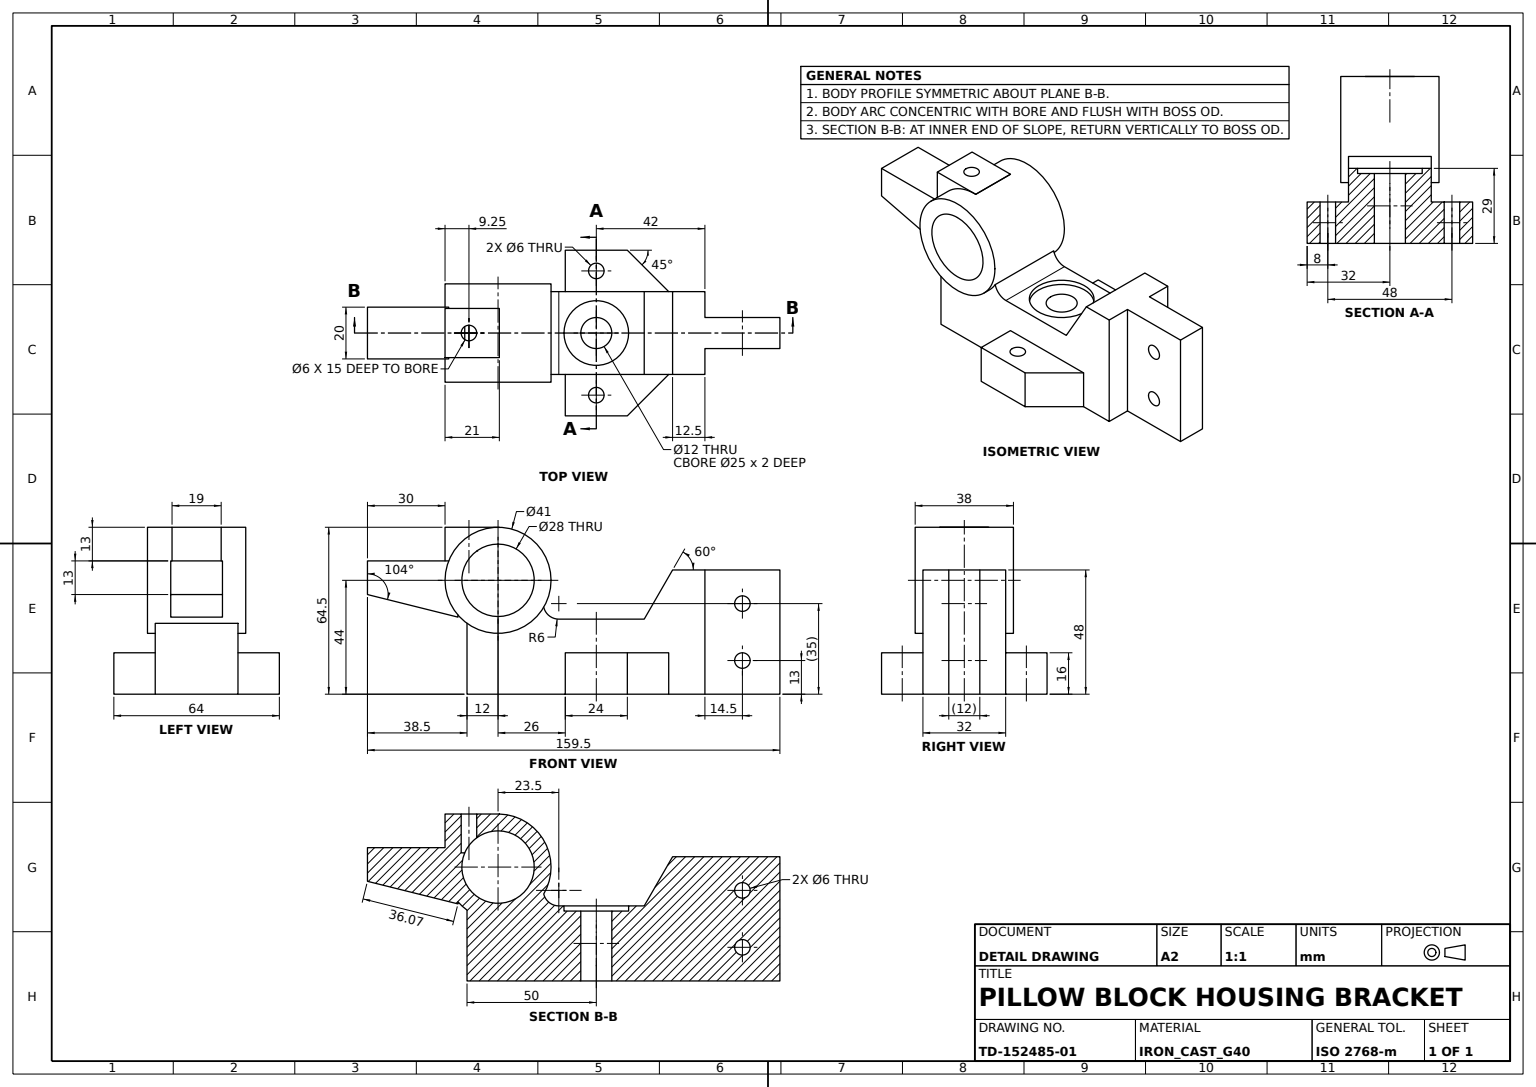
ISO-10303-21;
HEADER;
FILE_DESCRIPTION((''),'2;1');
FILE_NAME('','',(''),(''),'','','');
FILE_SCHEMA(('AUTOMOTIVE_DESIGN'));
ENDSEC;
DATA;
#1=APPLICATION_CONTEXT('');
#2=PRODUCT_CONTEXT('',#1,'mechanical');
#3=PRODUCT('','','',(#2));
#4=PRODUCT_DEFINITION_FORMATION('','',#3);
#5=PRODUCT_DEFINITION_CONTEXT('',#1,'design');
#6=PRODUCT_DEFINITION('','',#4,#5);
#7=PRODUCT_DEFINITION_SHAPE('','',#6);
#8=(LENGTH_UNIT()NAMED_UNIT(*)SI_UNIT(.MILLI.,.METRE.));
#9=(NAMED_UNIT(*)PLANE_ANGLE_UNIT()SI_UNIT($,.RADIAN.));
#10=(NAMED_UNIT(*)SI_UNIT($,.STERADIAN.)SOLID_ANGLE_UNIT());
#11=UNCERTAINTY_MEASURE_WITH_UNIT(LENGTH_MEASURE(0.005),#8,'distance_accuracy_value','');
#12=(GEOMETRIC_REPRESENTATION_CONTEXT(3)GLOBAL_UNCERTAINTY_ASSIGNED_CONTEXT((#11))GLOBAL_UNIT_ASSIGNED_CONTEXT((#8,#9,#10))REPRESENTATION_CONTEXT('',''));
#13=CARTESIAN_POINT('',(-60.5,16.,3.37923));
#14=VERTEX_POINT('',#13);
#15=CARTESIAN_POINT('',(-60.5,-16.,3.37923));
#16=VERTEX_POINT('',#15);
#17=CARTESIAN_POINT('',(-60.5,-19.,3.37923));
#18=DIRECTION('',(0.,1.,0.));
#19=VECTOR('',#18,1000.);
#20=LINE('',#17,#19);
#21=EDGE_CURVE('',#14,#16,#20,.F.);
#22=ORIENTED_EDGE('',*,*,#21,.T.);
#23=CARTESIAN_POINT('',(-30.834251,-16.,9.599457));
#24=VERTEX_POINT('',#23);
#25=CARTESIAN_POINT('',(-48.5,-16.,20.));
#26=DIRECTION('',(0.,-1.,0.));
#27=DIRECTION('',(0.,0.,-1.));
#28=AXIS2_PLACEMENT_3D('',#25,#26,#27);
#29=CIRCLE('',#28,20.5);
#30=EDGE_CURVE('',#24,#16,#29,.F.);
#31=ORIENTED_EDGE('',*,*,#30,.F.);
#32=CARTESIAN_POINT('',(-30.834251,16.,9.599457));
#33=VERTEX_POINT('',#32);
#34=CARTESIAN_POINT('',(-30.834251,0.,9.599457));
#35=LINE('',#34,#19);
#36=EDGE_CURVE('',#24,#33,#35,.T.);
#37=ORIENTED_EDGE('',*,*,#36,.T.);
#38=CARTESIAN_POINT('',(-48.5,16.,20.));
#39=DIRECTION('',(0.,0.,1.));
#40=AXIS2_PLACEMENT_3D('',#38,#18,#39);
#41=CIRCLE('',#40,20.5);
#42=EDGE_CURVE('',#14,#33,#41,.F.);
#43=ORIENTED_EDGE('',*,*,#42,.F.);
#44=EDGE_LOOP('',(#22,#31,#37,#43));
#45=FACE_BOUND('',#44,.T.);
#46=CARTESIAN_POINT('',(-28.,-19.,20.));
#47=VERTEX_POINT('',#46);
#48=CARTESIAN_POINT('',(-48.5,-19.,20.));
#49=DIRECTION('',(1.,0.,0.));
#50=AXIS2_PLACEMENT_3D('',#48,#26,#49);
#51=CIRCLE('',#50,20.5);
#52=EDGE_CURVE('',#47,#47,#51,.T.);
#53=ORIENTED_EDGE('',*,*,#52,.F.);
#54=EDGE_LOOP('',(#53));
#55=FACE_BOUND('',#54,.T.);
#56=CARTESIAN_POINT('',(-28.,19.,20.));
#57=VERTEX_POINT('',#56);
#58=CARTESIAN_POINT('',(-48.5,19.,20.));
#59=AXIS2_PLACEMENT_3D('',#58,#26,#49);
#60=CIRCLE('',#59,20.5);
#61=EDGE_CURVE('',#57,#57,#60,.T.);
#62=ORIENTED_EDGE('',*,*,#61,.T.);
#63=EDGE_LOOP('',(#62));
#64=FACE_BOUND('',#63,.T.);
#65=CARTESIAN_POINT('',(-67.578784,-10.,27.5));
#66=VERTEX_POINT('',#65);
#67=CARTESIAN_POINT('',(-67.578784,-9.5,27.5));
#68=VERTEX_POINT('',#67);
#69=CARTESIAN_POINT('',(-67.578784,-19.,27.5));
#70=LINE('',#69,#19);
#71=EDGE_CURVE('',#66,#68,#70,.T.);
#72=ORIENTED_EDGE('',*,*,#71,.F.);
#73=CARTESIAN_POINT('',(-64.,-10.,6.583592));
#74=VERTEX_POINT('',#73);
#75=CARTESIAN_POINT('',(-48.5,-10.,20.));
#76=AXIS2_PLACEMENT_3D('',#75,#18,#39);
#77=CIRCLE('',#76,20.5);
#78=EDGE_CURVE('',#74,#66,#77,.T.);
#79=ORIENTED_EDGE('',*,*,#78,.F.);
#80=CARTESIAN_POINT('',(-64.,10.,6.583592));
#81=VERTEX_POINT('',#80);
#82=CARTESIAN_POINT('',(-64.,-19.,6.583592));
#83=LINE('',#82,#19);
#84=EDGE_CURVE('',#81,#74,#83,.F.);
#85=ORIENTED_EDGE('',*,*,#84,.F.);
#86=CARTESIAN_POINT('',(-67.578784,10.,27.5));
#87=VERTEX_POINT('',#86);
#88=CARTESIAN_POINT('',(-48.5,10.,20.));
#89=AXIS2_PLACEMENT_3D('',#88,#18,#39);
#90=CIRCLE('',#89,20.5);
#91=EDGE_CURVE('',#81,#87,#90,.T.);
#92=ORIENTED_EDGE('',*,*,#91,.T.);
#93=CARTESIAN_POINT('',(-67.578784,9.5,27.5));
#94=VERTEX_POINT('',#93);
#95=EDGE_CURVE('',#94,#87,#70,.T.);
#96=ORIENTED_EDGE('',*,*,#95,.F.);
#97=CARTESIAN_POINT('',(-48.5,9.5,40.5));
#98=VERTEX_POINT('',#97);
#99=CARTESIAN_POINT('',(-48.5,9.5,20.));
#100=AXIS2_PLACEMENT_3D('',#99,#18,#39);
#101=CIRCLE('',#100,20.5);
#102=EDGE_CURVE('',#94,#98,#101,.T.);
#103=ORIENTED_EDGE('',*,*,#102,.T.);
#104=CARTESIAN_POINT('',(-48.,9.5,40.493902));
#105=VERTEX_POINT('',#104);
#106=EDGE_CURVE('',#98,#105,#101,.T.);
#107=ORIENTED_EDGE('',*,*,#106,.T.);
#108=CARTESIAN_POINT('',(-48.,-9.5,40.493902));
#109=VERTEX_POINT('',#108);
#110=CARTESIAN_POINT('',(-48.,-19.,40.493902));
#111=LINE('',#110,#19);
#112=EDGE_CURVE('',#105,#109,#111,.F.);
#113=ORIENTED_EDGE('',*,*,#112,.T.);
#114=CARTESIAN_POINT('',(-48.5,-9.5,40.5));
#115=VERTEX_POINT('',#114);
#116=CARTESIAN_POINT('',(-48.5,-9.5,20.));
#117=AXIS2_PLACEMENT_3D('',#116,#18,#39);
#118=CIRCLE('',#117,20.5);
#119=EDGE_CURVE('',#115,#109,#118,.T.);
#120=ORIENTED_EDGE('',*,*,#119,.F.);
#121=EDGE_CURVE('',#68,#115,#118,.T.);
#122=ORIENTED_EDGE('',*,*,#121,.F.);
#123=EDGE_LOOP('',(#72,#79,#85,#92,#96,#103,#107,#113,#120,#122));
#124=FACE_BOUND('',#123,.T.);
#125=AXIS2_PLACEMENT_3D('',#48,#18,#39);
#126=CYLINDRICAL_SURFACE('',#125,20.5);
#127=ADVANCED_FACE('',(#45,#55,#64,#124),#126,.T.);
#128=CARTESIAN_POINT('',(-22.5,16.,-24.));
#129=VERTEX_POINT('',#128);
#130=CARTESIAN_POINT('',(-22.5,16.,-8.));
#131=VERTEX_POINT('',#130);
#132=VECTOR('',#39,1000.);
#133=LINE('',#128,#132);
#134=EDGE_CURVE('',#129,#131,#133,.T.);
#135=ORIENTED_EDGE('',*,*,#134,.T.);
#136=CARTESIAN_POINT('',(-22.5,32.,-8.));
#137=VERTEX_POINT('',#136);
#138=VECTOR('',#26,1000.);
#139=LINE('',#136,#138);
#140=EDGE_CURVE('',#137,#131,#139,.T.);
#141=ORIENTED_EDGE('',*,*,#140,.F.);
#142=CARTESIAN_POINT('',(-22.5,32.,-24.));
#143=VERTEX_POINT('',#142);
#144=LINE('',#142,#132);
#145=EDGE_CURVE('',#143,#137,#144,.T.);
#146=ORIENTED_EDGE('',*,*,#145,.F.);
#147=LINE('',#142,#138);
#148=EDGE_CURVE('',#143,#129,#147,.T.);
#149=ORIENTED_EDGE('',*,*,#148,.T.);
#150=EDGE_LOOP('',(#135,#141,#146,#149));
#151=FACE_BOUND('',#150,.T.);
#152=DIRECTION('',(-1.,0.,0.));
#153=AXIS2_PLACEMENT_3D('',#142,#152,#26);
#154=PLANE('',#153);
#155=ADVANCED_FACE('',(#151),#154,.T.);
#156=CARTESIAN_POINT('',(-48.5,-19.,34.));
#157=VERTEX_POINT('',#156);
#158=CIRCLE('',#125,14.);
#159=EDGE_CURVE('',#157,#157,#158,.T.);
#160=ORIENTED_EDGE('',*,*,#159,.F.);
#161=EDGE_LOOP('',(#160));
#162=FACE_BOUND('',#161,.T.);
#163=CARTESIAN_POINT('',(-61.374393,-2.521118,25.5));
#164=VERTEX_POINT('',#163);
#165=CARTESIAN_POINT('',(-61.374393,2.521118,25.5));
#166=VERTEX_POINT('',#165);
#167=CARTESIAN_POINT('',(-61.084849,-2.707863,26.177764));
#168=CARTESIAN_POINT('',(-60.401421,-3.010301,27.486339));
#169=CARTESIAN_POINT('',(-59.021518,-3.045875,29.334769));
#170=CARTESIAN_POINT('',(-57.674961,-2.348709,30.602707));
#171=CARTESIAN_POINT('',(-56.899715,-1.143026,31.203678));
#172=CARTESIAN_POINT('',(-56.672943,-0.003656,31.366172));
#173=CARTESIAN_POINT('',(-56.898711,1.143364,31.204459));
#174=CARTESIAN_POINT('',(-57.67958,2.353835,30.59909));
#175=CARTESIAN_POINT('',(-59.028407,3.046836,29.326902));
#176=CARTESIAN_POINT('',(-60.40318,3.009307,27.482732));
#177=CARTESIAN_POINT('',(-61.085032,2.707745,26.177337));
#178=B_SPLINE_CURVE_WITH_KNOTS('',3,(#163,#167,#168,#169,#170,#171,#172,#173,#174,#175,#176,#177,#165),.UNSPECIFIED.,.F.,.F.,(4,1,1,1,1,1,1,1,1,1,4),(0.,0.002259018,0.004518035,0.006777053,0.007906562,0.009036071,0.010165579,0.011295088,0.013554106,0.015813124,0.018072141),.UNSPECIFIED.);
#179=EDGE_CURVE('',#164,#166,#178,.T.);
#180=ORIENTED_EDGE('',*,*,#179,.T.);
#181=CARTESIAN_POINT('',(-61.374393,-19.,25.5));
#182=LINE('',#181,#19);
#183=EDGE_CURVE('',#166,#164,#182,.F.);
#184=ORIENTED_EDGE('',*,*,#183,.T.);
#185=EDGE_LOOP('',(#180,#184));
#186=FACE_BOUND('',#185,.T.);
#187=CARTESIAN_POINT('',(-48.5,19.,6.));
#188=VERTEX_POINT('',#187);
#189=AXIS2_PLACEMENT_3D('',#58,#26,#27);
#190=CIRCLE('',#189,14.);
#191=EDGE_CURVE('',#188,#188,#190,.T.);
#192=ORIENTED_EDGE('',*,*,#191,.F.);
#193=EDGE_LOOP('',(#192));
#194=FACE_BOUND('',#193,.T.);
#195=CYLINDRICAL_SURFACE('',#125,14.);
#196=ADVANCED_FACE('',(#162,#186,#194),#195,.F.);
#197=ORIENTED_EDGE('',*,*,#52,.T.);
#198=EDGE_LOOP('',(#197));
#199=FACE_BOUND('',#198,.T.);
#200=ORIENTED_EDGE('',*,*,#159,.T.);
#201=EDGE_LOOP('',(#200));
#202=FACE_BOUND('',#201,.T.);
#203=AXIS2_PLACEMENT_3D('',#48,#26,#27);
#204=PLANE('',#203);
#205=ADVANCED_FACE('',(#199,#202),#204,.T.);
#206=CARTESIAN_POINT('',(-23.,0.,3.));
#207=VERTEX_POINT('',#206);
#208=CARTESIAN_POINT('',(-10.5,0.,3.));
#209=AXIS2_PLACEMENT_3D('',#208,#27,#152);
#210=CIRCLE('',#209,12.5);
#211=EDGE_CURVE('',#207,#207,#210,.F.);
#212=ORIENTED_EDGE('',*,*,#211,.F.);
#213=EDGE_LOOP('',(#212));
#214=FACE_BOUND('',#213,.T.);
#215=CARTESIAN_POINT('',(-23.,0.,5.));
#216=VERTEX_POINT('',#215);
#217=CARTESIAN_POINT('',(-10.5,0.,5.));
#218=AXIS2_PLACEMENT_3D('',#217,#27,#152);
#219=CIRCLE('',#218,12.5);
#220=EDGE_CURVE('',#216,#216,#219,.T.);
#221=ORIENTED_EDGE('',*,*,#220,.F.);
#222=EDGE_LOOP('',(#221));
#223=FACE_BOUND('',#222,.T.);
#224=CYLINDRICAL_SURFACE('',#218,12.5);
#225=ADVANCED_FACE('',(#214,#223),#224,.F.);
#226=ORIENTED_EDGE('',*,*,#112,.F.);
#227=CARTESIAN_POINT('',(-48.,9.5,40.5));
#228=VERTEX_POINT('',#227);
#229=VECTOR('',#27,1000.);
#230=LINE('',#227,#229);
#231=EDGE_CURVE('',#228,#105,#230,.T.);
#232=ORIENTED_EDGE('',*,*,#231,.F.);
#233=CARTESIAN_POINT('',(-48.,-9.5,40.5));
#234=VERTEX_POINT('',#233);
#235=LINE('',#233,#19);
#236=EDGE_CURVE('',#234,#228,#235,.T.);
#237=ORIENTED_EDGE('',*,*,#236,.F.);
#238=LINE('',#233,#229);
#239=EDGE_CURVE('',#234,#109,#238,.T.);
#240=ORIENTED_EDGE('',*,*,#239,.T.);
#241=EDGE_LOOP('',(#226,#232,#237,#240));
#242=FACE_BOUND('',#241,.T.);
#243=AXIS2_PLACEMENT_3D('',#233,#49,#27);
#244=PLANE('',#243);
#245=ADVANCED_FACE('',(#242),#244,.T.);
#246=CARTESIAN_POINT('',(17.5,-16.,-24.));
#247=VERTEX_POINT('',#246);
#248=CARTESIAN_POINT('',(1.5,-32.,-24.));
#249=VERTEX_POINT('',#248);
#250=DIRECTION('',(-0.707106781,-0.707106781,0.));
#251=VECTOR('',#250,1000.);
#252=LINE('',#246,#251);
#253=EDGE_CURVE('',#247,#249,#252,.T.);
#254=ORIENTED_EDGE('',*,*,#253,.F.);
#255=CARTESIAN_POINT('',(17.5,-16.,-8.));
#256=VERTEX_POINT('',#255);
#257=LINE('',#246,#132);
#258=EDGE_CURVE('',#247,#256,#257,.T.);
#259=ORIENTED_EDGE('',*,*,#258,.T.);
#260=CARTESIAN_POINT('',(1.5,-32.,-8.));
#261=VERTEX_POINT('',#260);
#262=LINE('',#255,#251);
#263=EDGE_CURVE('',#256,#261,#262,.T.);
#264=ORIENTED_EDGE('',*,*,#263,.T.);
#265=LINE('',#248,#132);
#266=EDGE_CURVE('',#249,#261,#265,.T.);
#267=ORIENTED_EDGE('',*,*,#266,.F.);
#268=EDGE_LOOP('',(#254,#259,#264,#267));
#269=FACE_BOUND('',#268,.T.);
#270=DIRECTION('',(-0.707106781,0.707106781,0.));
#271=AXIS2_PLACEMENT_3D('',#246,#270,#250);
#272=PLANE('',#271);
#273=ADVANCED_FACE('',(#269),#272,.F.);
#274=CARTESIAN_POINT('',(-69.,-9.5,40.5));
#275=VERTEX_POINT('',#274);
#276=CARTESIAN_POINT('',(-69.,9.5,40.5));
#277=VERTEX_POINT('',#276);
#278=LINE('',#274,#19);
#279=EDGE_CURVE('',#275,#277,#278,.T.);
#280=ORIENTED_EDGE('',*,*,#279,.T.);
#281=CARTESIAN_POINT('',(-69.,9.5,27.5));
#282=VERTEX_POINT('',#281);
#283=CARTESIAN_POINT('',(-69.,9.5,20.));
#284=LINE('',#283,#132);
#285=EDGE_CURVE('',#282,#277,#284,.T.);
#286=ORIENTED_EDGE('',*,*,#285,.F.);
#287=CARTESIAN_POINT('',(-69.,-9.5,27.5));
#288=VERTEX_POINT('',#287);
#289=LINE('',#287,#138);
#290=EDGE_CURVE('',#282,#288,#289,.T.);
#291=ORIENTED_EDGE('',*,*,#290,.T.);
#292=CARTESIAN_POINT('',(-69.,-9.5,20.));
#293=LINE('',#292,#132);
#294=EDGE_CURVE('',#288,#275,#293,.T.);
#295=ORIENTED_EDGE('',*,*,#294,.T.);
#296=EDGE_LOOP('',(#280,#286,#291,#295));
#297=FACE_BOUND('',#296,.T.);
#298=AXIS2_PLACEMENT_3D('',#292,#152,#39);
#299=PLANE('',#298);
#300=ADVANCED_FACE('',(#297),#299,.T.);
#301=CARTESIAN_POINT('',(-99.,-10.,27.5));
#302=VERTEX_POINT('',#301);
#303=CARTESIAN_POINT('',(-64.,-10.,27.5));
#304=VECTOR('',#152,1000.);
#305=LINE('',#303,#304);
#306=EDGE_CURVE('',#66,#302,#305,.T.);
#307=ORIENTED_EDGE('',*,*,#306,.T.);
#308=CARTESIAN_POINT('',(-99.,-10.,14.5));
#309=VERTEX_POINT('',#308);
#310=LINE('',#301,#229);
#311=EDGE_CURVE('',#302,#309,#310,.T.);
#312=ORIENTED_EDGE('',*,*,#311,.T.);
#313=CARTESIAN_POINT('',(-64.,-10.,5.77352));
#314=VERTEX_POINT('',#313);
#315=DIRECTION('',(0.970295726,0.,-0.241921896));
#316=VECTOR('',#315,1000.);
#317=LINE('',#308,#316);
#318=EDGE_CURVE('',#309,#314,#317,.T.);
#319=ORIENTED_EDGE('',*,*,#318,.T.);
#320=LINE('',#313,#132);
#321=EDGE_CURVE('',#314,#74,#320,.T.);
#322=ORIENTED_EDGE('',*,*,#321,.T.);
#323=ORIENTED_EDGE('',*,*,#78,.T.);
#324=EDGE_LOOP('',(#307,#312,#319,#322,#323));
#325=FACE_BOUND('',#324,.T.);
#326=CARTESIAN_POINT('',(0.,-10.,0.));
#327=AXIS2_PLACEMENT_3D('',#326,#18,#39);
#328=PLANE('',#327);
#329=ADVANCED_FACE('',(#325),#328,.F.);
#330=ORIENTED_EDGE('',*,*,#21,.F.);
#331=CARTESIAN_POINT('',(-60.5,16.,-24.));
#332=VERTEX_POINT('',#331);
#333=LINE('',#331,#132);
#334=EDGE_CURVE('',#332,#14,#333,.T.);
#335=ORIENTED_EDGE('',*,*,#334,.F.);
#336=CARTESIAN_POINT('',(-60.5,-16.,-24.));
#337=VERTEX_POINT('',#336);
#338=LINE('',#336,#19);
#339=EDGE_CURVE('',#337,#332,#338,.T.);
#340=ORIENTED_EDGE('',*,*,#339,.F.);
#341=CARTESIAN_POINT('',(-60.5,-16.,24.));
#342=LINE('',#341,#229);
#343=EDGE_CURVE('',#16,#337,#342,.T.);
#344=ORIENTED_EDGE('',*,*,#343,.F.);
#345=EDGE_LOOP('',(#330,#335,#340,#344));
#346=FACE_BOUND('',#345,.T.);
#347=CARTESIAN_POINT('',(-60.5,0.,0.));
#348=AXIS2_PLACEMENT_3D('',#347,#49,#27);
#349=PLANE('',#348);
#350=ADVANCED_FACE('',(#346),#349,.F.);
#351=CARTESIAN_POINT('',(19.,-16.,24.));
#352=VERTEX_POINT('',#351);
#353=CARTESIAN_POINT('',(19.,16.,24.));
#354=VERTEX_POINT('',#353);
#355=CARTESIAN_POINT('',(19.,-60.5,24.));
#356=LINE('',#355,#19);
#357=EDGE_CURVE('',#352,#354,#356,.T.);
#358=ORIENTED_EDGE('',*,*,#357,.T.);
#359=CARTESIAN_POINT('',(8.030345,16.,5.));
#360=VERTEX_POINT('',#359);
#361=CARTESIAN_POINT('',(-21.65961,16.,-46.42451));
#362=DIRECTION('',(0.5,0.,0.866025404));
#363=VECTOR('',#362,1000.);
#364=LINE('',#361,#363);
#365=EDGE_CURVE('',#360,#354,#364,.T.);
#366=ORIENTED_EDGE('',*,*,#365,.F.);
#367=CARTESIAN_POINT('',(8.030345,-16.,5.));
#368=VERTEX_POINT('',#367);
#369=CARTESIAN_POINT('',(8.030345,-60.5,5.));
#370=LINE('',#369,#19);
#371=EDGE_CURVE('',#360,#368,#370,.F.);
#372=ORIENTED_EDGE('',*,*,#371,.T.);
#373=CARTESIAN_POINT('',(-0.875,-16.,-10.42451));
#374=DIRECTION('',(-0.5,0.,-0.866025404));
#375=VECTOR('',#374,1000.);
#376=LINE('',#373,#375);
#377=EDGE_CURVE('',#352,#368,#376,.T.);
#378=ORIENTED_EDGE('',*,*,#377,.F.);
#379=EDGE_LOOP('',(#358,#366,#372,#378));
#380=FACE_BOUND('',#379,.T.);
#381=DIRECTION('',(-0.866025404,0.,0.5));
#382=AXIS2_PLACEMENT_3D('',#369,#381,#362);
#383=PLANE('',#382);
#384=ADVANCED_FACE('',(#380),#383,.T.);
#385=CARTESIAN_POINT('',(-13.5,-24.,-24.));
#386=VERTEX_POINT('',#385);
#387=CARTESIAN_POINT('',(-10.5,-24.,-24.));
#388=AXIS2_PLACEMENT_3D('',#387,#27,#152);
#389=CIRCLE('',#388,3.);
#390=EDGE_CURVE('',#386,#386,#389,.T.);
#391=ORIENTED_EDGE('',*,*,#390,.T.);
#392=EDGE_LOOP('',(#391));
#393=FACE_BOUND('',#392,.T.);
#394=CARTESIAN_POINT('',(-13.5,-24.,-8.));
#395=VERTEX_POINT('',#394);
#396=CARTESIAN_POINT('',(-10.5,-24.,-8.));
#397=AXIS2_PLACEMENT_3D('',#396,#27,#152);
#398=CIRCLE('',#397,3.);
#399=EDGE_CURVE('',#395,#395,#398,.T.);
#400=ORIENTED_EDGE('',*,*,#399,.F.);
#401=EDGE_LOOP('',(#400));
#402=FACE_BOUND('',#401,.T.);
#403=CYLINDRICAL_SURFACE('',#397,3.);
#404=ADVANCED_FACE('',(#393,#402),#403,.F.);
#405=CARTESIAN_POINT('',(-62.748365,0.,40.5));
#406=VERTEX_POINT('',#405);
#407=CARTESIAN_POINT('',(-59.748365,0.,40.5));
#408=AXIS2_PLACEMENT_3D('',#407,#27,#152);
#409=CIRCLE('',#408,3.);
#410=EDGE_CURVE('',#406,#406,#409,.T.);
#411=ORIENTED_EDGE('',*,*,#410,.F.);
#412=EDGE_LOOP('',(#411));
#413=FACE_BOUND('',#412,.T.);
#414=CARTESIAN_POINT('',(-59.748365,0.,25.5));
#415=AXIS2_PLACEMENT_3D('',#414,#27,#152);
#416=CIRCLE('',#415,3.);
#417=EDGE_CURVE('',#166,#164,#416,.F.);
#418=ORIENTED_EDGE('',*,*,#417,.F.);
#419=ORIENTED_EDGE('',*,*,#179,.F.);
#420=EDGE_LOOP('',(#418,#419));
#421=FACE_BOUND('',#420,.T.);
#422=CYLINDRICAL_SURFACE('',#408,3.);
#423=ADVANCED_FACE('',(#413,#421),#422,.F.);
#424=ORIENTED_EDGE('',*,*,#399,.T.);
#425=EDGE_LOOP('',(#424));
#426=FACE_BOUND('',#425,.T.);
#427=CARTESIAN_POINT('',(-22.5,-32.,-8.));
#428=VERTEX_POINT('',#427);
#429=LINE('',#260,#304);
#430=EDGE_CURVE('',#261,#428,#429,.T.);
#431=ORIENTED_EDGE('',*,*,#430,.F.);
#432=ORIENTED_EDGE('',*,*,#263,.F.);
#433=CARTESIAN_POINT('',(-22.5,-16.,-8.));
#434=VERTEX_POINT('',#433);
#435=VECTOR('',#49,1000.);
#436=LINE('',#433,#435);
#437=EDGE_CURVE('',#434,#256,#436,.T.);
#438=ORIENTED_EDGE('',*,*,#437,.F.);
#439=LINE('',#427,#19);
#440=EDGE_CURVE('',#428,#434,#439,.T.);
#441=ORIENTED_EDGE('',*,*,#440,.F.);
#442=EDGE_LOOP('',(#431,#432,#438,#441));
#443=FACE_BOUND('',#442,.T.);
#444=CARTESIAN_POINT('',(0.,0.,-8.));
#445=AXIS2_PLACEMENT_3D('',#444,#27,#152);
#446=PLANE('',#445);
#447=ADVANCED_FACE('',(#426,#443),#446,.F.);
#448=ORIENTED_EDGE('',*,*,#430,.T.);
#449=CARTESIAN_POINT('',(-22.5,-32.,-24.));
#450=VERTEX_POINT('',#449);
#451=LINE('',#449,#132);
#452=EDGE_CURVE('',#450,#428,#451,.T.);
#453=ORIENTED_EDGE('',*,*,#452,.F.);
#454=LINE('',#248,#304);
#455=EDGE_CURVE('',#249,#450,#454,.T.);
#456=ORIENTED_EDGE('',*,*,#455,.F.);
#457=ORIENTED_EDGE('',*,*,#266,.T.);
#458=EDGE_LOOP('',(#448,#453,#456,#457));
#459=FACE_BOUND('',#458,.T.);
#460=AXIS2_PLACEMENT_3D('',#248,#18,#39);
#461=PLANE('',#460);
#462=ADVANCED_FACE('',(#459),#461,.F.);
#463=CARTESIAN_POINT('',(43.,-6.,-11.));
#464=VERTEX_POINT('',#463);
#465=CARTESIAN_POINT('',(46.,-6.,-11.));
#466=AXIS2_PLACEMENT_3D('',#465,#18,#152);
#467=CIRCLE('',#466,3.);
#468=EDGE_CURVE('',#464,#464,#467,.T.);
#469=ORIENTED_EDGE('',*,*,#468,.F.);
#470=EDGE_LOOP('',(#469));
#471=FACE_BOUND('',#470,.T.);
#472=CARTESIAN_POINT('',(43.,6.,-11.));
#473=VERTEX_POINT('',#472);
#474=CARTESIAN_POINT('',(46.,6.,-11.));
#475=AXIS2_PLACEMENT_3D('',#474,#18,#152);
#476=CIRCLE('',#475,3.);
#477=EDGE_CURVE('',#473,#473,#476,.T.);
#478=ORIENTED_EDGE('',*,*,#477,.T.);
#479=EDGE_LOOP('',(#478));
#480=FACE_BOUND('',#479,.T.);
#481=CYLINDRICAL_SURFACE('',#466,3.);
#482=ADVANCED_FACE('',(#471,#480),#481,.F.);
#483=CARTESIAN_POINT('',(-99.,10.,27.5));
#484=VERTEX_POINT('',#483);
#485=LINE('',#301,#19);
#486=EDGE_CURVE('',#302,#484,#485,.T.);
#487=ORIENTED_EDGE('',*,*,#486,.T.);
#488=CARTESIAN_POINT('',(-99.,10.,14.5));
#489=VERTEX_POINT('',#488);
#490=LINE('',#483,#229);
#491=EDGE_CURVE('',#484,#489,#490,.T.);
#492=ORIENTED_EDGE('',*,*,#491,.T.);
#493=LINE('',#308,#19);
#494=EDGE_CURVE('',#309,#489,#493,.T.);
#495=ORIENTED_EDGE('',*,*,#494,.F.);
#496=ORIENTED_EDGE('',*,*,#311,.F.);
#497=EDGE_LOOP('',(#487,#492,#495,#496));
#498=FACE_BOUND('',#497,.T.);
#499=AXIS2_PLACEMENT_3D('',#301,#49,#27);
#500=PLANE('',#499);
#501=ADVANCED_FACE('',(#498),#500,.F.);
#502=CARTESIAN_POINT('',(-13.5,24.,-8.));
#503=VERTEX_POINT('',#502);
#504=CARTESIAN_POINT('',(-10.5,24.,-8.));
#505=AXIS2_PLACEMENT_3D('',#504,#27,#152);
#506=CIRCLE('',#505,3.);
#507=EDGE_CURVE('',#503,#503,#506,.T.);
#508=ORIENTED_EDGE('',*,*,#507,.T.);
#509=EDGE_LOOP('',(#508));
#510=FACE_BOUND('',#509,.T.);
#511=CARTESIAN_POINT('',(17.5,16.,-8.));
#512=VERTEX_POINT('',#511);
#513=CARTESIAN_POINT('',(1.5,32.,-8.));
#514=VERTEX_POINT('',#513);
#515=VECTOR('',#270,1000.);
#516=LINE('',#511,#515);
#517=EDGE_CURVE('',#512,#514,#516,.T.);
#518=ORIENTED_EDGE('',*,*,#517,.T.);
#519=LINE('',#513,#304);
#520=EDGE_CURVE('',#514,#137,#519,.T.);
#521=ORIENTED_EDGE('',*,*,#520,.T.);
#522=ORIENTED_EDGE('',*,*,#140,.T.);
#523=LINE('',#130,#435);
#524=EDGE_CURVE('',#131,#512,#523,.T.);
#525=ORIENTED_EDGE('',*,*,#524,.T.);
#526=EDGE_LOOP('',(#518,#521,#522,#525));
#527=FACE_BOUND('',#526,.T.);
#528=AXIS2_PLACEMENT_3D('',#444,#39,#49);
#529=PLANE('',#528);
#530=ADVANCED_FACE('',(#510,#527),#529,.T.);
#531=ORIENTED_EDGE('',*,*,#520,.F.);
#532=CARTESIAN_POINT('',(1.5,32.,-24.));
#533=VERTEX_POINT('',#532);
#534=LINE('',#532,#132);
#535=EDGE_CURVE('',#533,#514,#534,.T.);
#536=ORIENTED_EDGE('',*,*,#535,.F.);
#537=LINE('',#532,#304);
#538=EDGE_CURVE('',#533,#143,#537,.T.);
#539=ORIENTED_EDGE('',*,*,#538,.T.);
#540=ORIENTED_EDGE('',*,*,#145,.T.);
#541=EDGE_LOOP('',(#531,#536,#539,#540));
#542=FACE_BOUND('',#541,.T.);
#543=AXIS2_PLACEMENT_3D('',#532,#18,#39);
#544=PLANE('',#543);
#545=ADVANCED_FACE('',(#542),#544,.T.);
#546=CARTESIAN_POINT('',(43.,-6.,11.));
#547=VERTEX_POINT('',#546);
#548=CARTESIAN_POINT('',(46.,-6.,11.));
#549=AXIS2_PLACEMENT_3D('',#548,#18,#152);
#550=CIRCLE('',#549,3.);
#551=EDGE_CURVE('',#547,#547,#550,.T.);
#552=ORIENTED_EDGE('',*,*,#551,.F.);
#553=EDGE_LOOP('',(#552));
#554=FACE_BOUND('',#553,.T.);
#555=CARTESIAN_POINT('',(43.,6.,11.));
#556=VERTEX_POINT('',#555);
#557=CARTESIAN_POINT('',(46.,6.,11.));
#558=AXIS2_PLACEMENT_3D('',#557,#18,#152);
#559=CIRCLE('',#558,3.);
#560=EDGE_CURVE('',#556,#556,#559,.T.);
#561=ORIENTED_EDGE('',*,*,#560,.T.);
#562=EDGE_LOOP('',(#561));
#563=FACE_BOUND('',#562,.T.);
#564=CYLINDRICAL_SURFACE('',#549,3.);
#565=ADVANCED_FACE('',(#554,#563),#564,.F.);
#566=CARTESIAN_POINT('',(-64.,10.,5.77352));
#567=VERTEX_POINT('',#566);
#568=LINE('',#313,#19);
#569=EDGE_CURVE('',#314,#567,#568,.T.);
#570=ORIENTED_EDGE('',*,*,#569,.T.);
#571=LINE('',#566,#132);
#572=EDGE_CURVE('',#567,#81,#571,.T.);
#573=ORIENTED_EDGE('',*,*,#572,.T.);
#574=ORIENTED_EDGE('',*,*,#84,.T.);
#575=ORIENTED_EDGE('',*,*,#321,.F.);
#576=EDGE_LOOP('',(#570,#573,#574,#575));
#577=FACE_BOUND('',#576,.T.);
#578=AXIS2_PLACEMENT_3D('',#313,#152,#39);
#579=PLANE('',#578);
#580=ADVANCED_FACE('',(#577),#579,.F.);
#581=ORIENTED_EDGE('',*,*,#390,.F.);
#582=EDGE_LOOP('',(#581));
#583=FACE_BOUND('',#582,.T.);
#584=ORIENTED_EDGE('',*,*,#538,.F.);
#585=CARTESIAN_POINT('',(17.5,16.,-24.));
#586=VERTEX_POINT('',#585);
#587=LINE('',#585,#515);
#588=EDGE_CURVE('',#586,#533,#587,.T.);
#589=ORIENTED_EDGE('',*,*,#588,.F.);
#590=CARTESIAN_POINT('',(31.5,16.,-24.));
#591=VERTEX_POINT('',#590);
#592=LINE('',#331,#435);
#593=EDGE_CURVE('',#586,#591,#592,.T.);
#594=ORIENTED_EDGE('',*,*,#593,.T.);
#595=CARTESIAN_POINT('',(31.5,6.,-24.));
#596=VERTEX_POINT('',#595);
#597=CARTESIAN_POINT('',(31.5,-16.,-24.));
#598=LINE('',#597,#138);
#599=EDGE_CURVE('',#591,#596,#598,.T.);
#600=ORIENTED_EDGE('',*,*,#599,.T.);
#601=CARTESIAN_POINT('',(60.5,6.,-24.));
#602=VERTEX_POINT('',#601);
#603=CARTESIAN_POINT('',(-60.5,6.,-24.));
#604=LINE('',#603,#435);
#605=EDGE_CURVE('',#596,#602,#604,.T.);
#606=ORIENTED_EDGE('',*,*,#605,.T.);
#607=CARTESIAN_POINT('',(60.5,-6.,-24.));
#608=VERTEX_POINT('',#607);
#609=CARTESIAN_POINT('',(60.5,-16.,-24.));
#610=LINE('',#609,#19);
#611=EDGE_CURVE('',#608,#602,#610,.T.);
#612=ORIENTED_EDGE('',*,*,#611,.F.);
#613=CARTESIAN_POINT('',(31.5,-6.,-24.));
#614=VERTEX_POINT('',#613);
#615=CARTESIAN_POINT('',(-60.5,-6.,-24.));
#616=LINE('',#615,#435);
#617=EDGE_CURVE('',#614,#608,#616,.T.);
#618=ORIENTED_EDGE('',*,*,#617,.F.);
#619=VERTEX_POINT('',#597);
#620=LINE('',#597,#19);
#621=EDGE_CURVE('',#619,#614,#620,.T.);
#622=ORIENTED_EDGE('',*,*,#621,.F.);
#623=LINE('',#336,#435);
#624=EDGE_CURVE('',#247,#619,#623,.T.);
#625=ORIENTED_EDGE('',*,*,#624,.F.);
#626=ORIENTED_EDGE('',*,*,#253,.T.);
#627=ORIENTED_EDGE('',*,*,#455,.T.);
#628=CARTESIAN_POINT('',(-22.5,-16.,-24.));
#629=VERTEX_POINT('',#628);
#630=LINE('',#449,#19);
#631=EDGE_CURVE('',#450,#629,#630,.T.);
#632=ORIENTED_EDGE('',*,*,#631,.T.);
#633=EDGE_CURVE('',#337,#629,#623,.T.);
#634=ORIENTED_EDGE('',*,*,#633,.F.);
#635=ORIENTED_EDGE('',*,*,#339,.T.);
#636=EDGE_CURVE('',#332,#129,#592,.T.);
#637=ORIENTED_EDGE('',*,*,#636,.T.);
#638=ORIENTED_EDGE('',*,*,#148,.F.);
#639=EDGE_LOOP('',(#584,#589,#594,#600,#606,#612,#618,#622,#625,#626,#627,#632,#634,#635,#637,#638));
#640=FACE_BOUND('',#639,.T.);
#641=CARTESIAN_POINT('',(-13.5,24.,-24.));
#642=VERTEX_POINT('',#641);
#643=CARTESIAN_POINT('',(-10.5,24.,-24.));
#644=AXIS2_PLACEMENT_3D('',#643,#27,#152);
#645=CIRCLE('',#644,3.);
#646=EDGE_CURVE('',#642,#642,#645,.T.);
#647=ORIENTED_EDGE('',*,*,#646,.F.);
#648=EDGE_LOOP('',(#647));
#649=FACE_BOUND('',#648,.T.);
#650=CARTESIAN_POINT('',(-16.5,0.,-24.));
#651=VERTEX_POINT('',#650);
#652=CARTESIAN_POINT('',(-10.5,0.,-24.));
#653=AXIS2_PLACEMENT_3D('',#652,#27,#152);
#654=CIRCLE('',#653,6.);
#655=EDGE_CURVE('',#651,#651,#654,.T.);
#656=ORIENTED_EDGE('',*,*,#655,.F.);
#657=EDGE_LOOP('',(#656));
#658=FACE_BOUND('',#657,.T.);
#659=AXIS2_PLACEMENT_3D('',#336,#27,#152);
#660=PLANE('',#659);
#661=ADVANCED_FACE('',(#583,#640,#649,#658),#660,.T.);
#662=ORIENTED_EDGE('',*,*,#294,.F.);
#663=CARTESIAN_POINT('',(0.,-9.5,27.5));
#664=LINE('',#663,#304);
#665=EDGE_CURVE('',#68,#288,#664,.T.);
#666=ORIENTED_EDGE('',*,*,#665,.F.);
#667=ORIENTED_EDGE('',*,*,#121,.T.);
#668=LINE('',#274,#435);
#669=EDGE_CURVE('',#275,#115,#668,.T.);
#670=ORIENTED_EDGE('',*,*,#669,.F.);
#671=EDGE_LOOP('',(#662,#666,#667,#670));
#672=FACE_BOUND('',#671,.T.);
#673=CARTESIAN_POINT('',(0.,-9.5,0.));
#674=AXIS2_PLACEMENT_3D('',#673,#18,#39);
#675=PLANE('',#674);
#676=ADVANCED_FACE('',(#672),#675,.F.);
#677=ORIENTED_EDGE('',*,*,#357,.F.);
#678=CARTESIAN_POINT('',(31.5,-16.,24.));
#679=VERTEX_POINT('',#678);
#680=LINE('',#341,#435);
#681=EDGE_CURVE('',#352,#679,#680,.T.);
#682=ORIENTED_EDGE('',*,*,#681,.T.);
#683=CARTESIAN_POINT('',(31.5,-6.,24.));
#684=VERTEX_POINT('',#683);
#685=CARTESIAN_POINT('',(31.5,16.,24.));
#686=LINE('',#685,#138);
#687=EDGE_CURVE('',#684,#679,#686,.T.);
#688=ORIENTED_EDGE('',*,*,#687,.F.);
#689=CARTESIAN_POINT('',(60.5,-6.,24.));
#690=VERTEX_POINT('',#689);
#691=CARTESIAN_POINT('',(-60.5,-6.,24.));
#692=LINE('',#691,#304);
#693=EDGE_CURVE('',#690,#684,#692,.T.);
#694=ORIENTED_EDGE('',*,*,#693,.F.);
#695=CARTESIAN_POINT('',(60.5,6.,24.));
#696=VERTEX_POINT('',#695);
#697=CARTESIAN_POINT('',(60.5,16.,24.));
#698=LINE('',#697,#138);
#699=EDGE_CURVE('',#696,#690,#698,.T.);
#700=ORIENTED_EDGE('',*,*,#699,.F.);
#701=CARTESIAN_POINT('',(31.5,6.,24.));
#702=VERTEX_POINT('',#701);
#703=CARTESIAN_POINT('',(-60.5,6.,24.));
#704=LINE('',#703,#304);
#705=EDGE_CURVE('',#696,#702,#704,.T.);
#706=ORIENTED_EDGE('',*,*,#705,.T.);
#707=VERTEX_POINT('',#685);
#708=LINE('',#685,#19);
#709=EDGE_CURVE('',#702,#707,#708,.T.);
#710=ORIENTED_EDGE('',*,*,#709,.T.);
#711=CARTESIAN_POINT('',(-60.5,16.,24.));
#712=LINE('',#711,#435);
#713=EDGE_CURVE('',#354,#707,#712,.T.);
#714=ORIENTED_EDGE('',*,*,#713,.F.);
#715=EDGE_LOOP('',(#677,#682,#688,#694,#700,#706,#710,#714));
#716=FACE_BOUND('',#715,.T.);
#717=AXIS2_PLACEMENT_3D('',#711,#39,#49);
#718=PLANE('',#717);
#719=ADVANCED_FACE('',(#716),#718,.T.);
#720=ORIENTED_EDGE('',*,*,#560,.F.);
#721=EDGE_LOOP('',(#720));
#722=FACE_BOUND('',#721,.T.);
#723=ORIENTED_EDGE('',*,*,#477,.F.);
#724=EDGE_LOOP('',(#723));
#725=FACE_BOUND('',#724,.T.);
#726=CARTESIAN_POINT('',(60.5,6.,0.));
#727=LINE('',#726,#132);
#728=EDGE_CURVE('',#602,#696,#727,.T.);
#729=ORIENTED_EDGE('',*,*,#728,.F.);
#730=ORIENTED_EDGE('',*,*,#605,.F.);
#731=CARTESIAN_POINT('',(31.5,6.,60.5));
#732=LINE('',#731,#229);
#733=EDGE_CURVE('',#596,#702,#732,.F.);
#734=ORIENTED_EDGE('',*,*,#733,.T.);
#735=ORIENTED_EDGE('',*,*,#705,.F.);
#736=EDGE_LOOP('',(#729,#730,#734,#735));
#737=FACE_BOUND('',#736,.T.);
#738=AXIS2_PLACEMENT_3D('',#731,#18,#152);
#739=PLANE('',#738);
#740=ADVANCED_FACE('',(#722,#725,#737),#739,.T.);
#741=CARTESIAN_POINT('',(0.,9.5,27.5));
#742=LINE('',#741,#304);
#743=EDGE_CURVE('',#94,#282,#742,.T.);
#744=ORIENTED_EDGE('',*,*,#743,.T.);
#745=ORIENTED_EDGE('',*,*,#285,.T.);
#746=LINE('',#276,#435);
#747=EDGE_CURVE('',#277,#98,#746,.T.);
#748=ORIENTED_EDGE('',*,*,#747,.T.);
#749=ORIENTED_EDGE('',*,*,#102,.F.);
#750=EDGE_LOOP('',(#744,#745,#748,#749));
#751=FACE_BOUND('',#750,.T.);
#752=CARTESIAN_POINT('',(0.,9.5,0.));
#753=AXIS2_PLACEMENT_3D('',#752,#18,#39);
#754=PLANE('',#753);
#755=ADVANCED_FACE('',(#751),#754,.T.);
#756=LINE('',#628,#132);
#757=EDGE_CURVE('',#629,#434,#756,.T.);
#758=ORIENTED_EDGE('',*,*,#757,.T.);
#759=ORIENTED_EDGE('',*,*,#437,.T.);
#760=ORIENTED_EDGE('',*,*,#258,.F.);
#761=ORIENTED_EDGE('',*,*,#624,.T.);
#762=CARTESIAN_POINT('',(31.5,-16.,60.5));
#763=LINE('',#762,#229);
#764=EDGE_CURVE('',#619,#679,#763,.F.);
#765=ORIENTED_EDGE('',*,*,#764,.T.);
#766=ORIENTED_EDGE('',*,*,#681,.F.);
#767=ORIENTED_EDGE('',*,*,#377,.T.);
#768=CARTESIAN_POINT('',(-25.,-16.,5.));
#769=VERTEX_POINT('',#768);
#770=CARTESIAN_POINT('',(-60.5,-16.,5.));
#771=LINE('',#770,#304);
#772=EDGE_CURVE('',#368,#769,#771,.T.);
#773=ORIENTED_EDGE('',*,*,#772,.T.);
#774=CARTESIAN_POINT('',(-25.,-16.,11.));
#775=AXIS2_PLACEMENT_3D('',#774,#26,#27);
#776=CIRCLE('',#775,6.);
#777=EDGE_CURVE('',#769,#24,#776,.F.);
#778=ORIENTED_EDGE('',*,*,#777,.T.);
#779=ORIENTED_EDGE('',*,*,#30,.T.);
#780=ORIENTED_EDGE('',*,*,#343,.T.);
#781=ORIENTED_EDGE('',*,*,#633,.T.);
#782=EDGE_LOOP('',(#758,#759,#760,#761,#765,#766,#767,#773,#778,#779,#780,#781));
#783=FACE_BOUND('',#782,.T.);
#784=AXIS2_PLACEMENT_3D('',#341,#26,#27);
#785=PLANE('',#784);
#786=ADVANCED_FACE('',(#783),#785,.T.);
#787=ORIENTED_EDGE('',*,*,#95,.T.);
#788=CARTESIAN_POINT('',(-64.,10.,27.5));
#789=LINE('',#788,#304);
#790=EDGE_CURVE('',#87,#484,#789,.T.);
#791=ORIENTED_EDGE('',*,*,#790,.T.);
#792=ORIENTED_EDGE('',*,*,#486,.F.);
#793=ORIENTED_EDGE('',*,*,#306,.F.);
#794=ORIENTED_EDGE('',*,*,#71,.T.);
#795=ORIENTED_EDGE('',*,*,#665,.T.);
#796=ORIENTED_EDGE('',*,*,#290,.F.);
#797=ORIENTED_EDGE('',*,*,#743,.F.);
#798=EDGE_LOOP('',(#787,#791,#792,#793,#794,#795,#796,#797));
#799=FACE_BOUND('',#798,.T.);
#800=AXIS2_PLACEMENT_3D('',#303,#27,#152);
#801=PLANE('',#800);
#802=ADVANCED_FACE('',(#799),#801,.F.);
#803=ORIENTED_EDGE('',*,*,#764,.F.);
#804=ORIENTED_EDGE('',*,*,#621,.T.);
#805=CARTESIAN_POINT('',(31.5,-6.,60.5));
#806=LINE('',#805,#229);
#807=EDGE_CURVE('',#614,#684,#806,.F.);
#808=ORIENTED_EDGE('',*,*,#807,.T.);
#809=ORIENTED_EDGE('',*,*,#687,.T.);
#810=EDGE_LOOP('',(#803,#804,#808,#809));
#811=FACE_BOUND('',#810,.T.);
#812=AXIS2_PLACEMENT_3D('',#762,#152,#39);
#813=PLANE('',#812);
#814=ADVANCED_FACE('',(#811),#813,.F.);
#815=ORIENTED_EDGE('',*,*,#452,.T.);
#816=ORIENTED_EDGE('',*,*,#440,.T.);
#817=ORIENTED_EDGE('',*,*,#757,.F.);
#818=ORIENTED_EDGE('',*,*,#631,.F.);
#819=EDGE_LOOP('',(#815,#816,#817,#818));
#820=FACE_BOUND('',#819,.T.);
#821=AXIS2_PLACEMENT_3D('',#449,#49,#18);
#822=PLANE('',#821);
#823=ADVANCED_FACE('',(#820),#822,.F.);
#824=ORIENTED_EDGE('',*,*,#239,.F.);
#825=EDGE_CURVE('',#115,#234,#668,.T.);
#826=ORIENTED_EDGE('',*,*,#825,.F.);
#827=ORIENTED_EDGE('',*,*,#119,.T.);
#828=EDGE_LOOP('',(#824,#826,#827));
#829=FACE_BOUND('',#828,.T.);
#830=ADVANCED_FACE('',(#829),#675,.F.);
#831=ORIENTED_EDGE('',*,*,#535,.T.);
#832=ORIENTED_EDGE('',*,*,#517,.F.);
#833=LINE('',#585,#132);
#834=EDGE_CURVE('',#586,#512,#833,.T.);
#835=ORIENTED_EDGE('',*,*,#834,.F.);
#836=ORIENTED_EDGE('',*,*,#588,.T.);
#837=EDGE_LOOP('',(#831,#832,#835,#836));
#838=FACE_BOUND('',#837,.T.);
#839=DIRECTION('',(0.707106781,0.707106781,0.));
#840=AXIS2_PLACEMENT_3D('',#585,#839,#270);
#841=PLANE('',#840);
#842=ADVANCED_FACE('',(#838),#841,.T.);
#843=ORIENTED_EDGE('',*,*,#599,.F.);
#844=CARTESIAN_POINT('',(31.5,16.,60.5));
#845=LINE('',#844,#229);
#846=EDGE_CURVE('',#591,#707,#845,.F.);
#847=ORIENTED_EDGE('',*,*,#846,.T.);
#848=ORIENTED_EDGE('',*,*,#709,.F.);
#849=ORIENTED_EDGE('',*,*,#733,.F.);
#850=EDGE_LOOP('',(#843,#847,#848,#849));
#851=FACE_BOUND('',#850,.T.);
#852=AXIS2_PLACEMENT_3D('',#844,#49,#27);
#853=PLANE('',#852);
#854=ADVANCED_FACE('',(#851),#853,.T.);
#855=ORIENTED_EDGE('',*,*,#611,.T.);
#856=ORIENTED_EDGE('',*,*,#728,.T.);
#857=ORIENTED_EDGE('',*,*,#699,.T.);
#858=CARTESIAN_POINT('',(60.5,-6.,0.));
#859=LINE('',#858,#132);
#860=EDGE_CURVE('',#608,#690,#859,.T.);
#861=ORIENTED_EDGE('',*,*,#860,.F.);
#862=EDGE_LOOP('',(#855,#856,#857,#861));
#863=FACE_BOUND('',#862,.T.);
#864=CARTESIAN_POINT('',(60.5,0.,0.));
#865=AXIS2_PLACEMENT_3D('',#864,#49,#27);
#866=PLANE('',#865);
#867=ADVANCED_FACE('',(#863),#866,.T.);
#868=ORIENTED_EDGE('',*,*,#211,.T.);
#869=EDGE_LOOP('',(#868));
#870=FACE_BOUND('',#869,.T.);
#871=CARTESIAN_POINT('',(-16.5,0.,3.));
#872=VERTEX_POINT('',#871);
#873=CIRCLE('',#209,6.);
#874=EDGE_CURVE('',#872,#872,#873,.T.);
#875=ORIENTED_EDGE('',*,*,#874,.T.);
#876=EDGE_LOOP('',(#875));
#877=FACE_BOUND('',#876,.T.);
#878=PLANE('',#209);
#879=ADVANCED_FACE('',(#870,#877),#878,.F.);
#880=ORIENTED_EDGE('',*,*,#220,.T.);
#881=EDGE_LOOP('',(#880));
#882=FACE_BOUND('',#881,.T.);
#883=ORIENTED_EDGE('',*,*,#371,.F.);
#884=CARTESIAN_POINT('',(-25.,16.,5.));
#885=VERTEX_POINT('',#884);
#886=CARTESIAN_POINT('',(-60.5,16.,5.));
#887=LINE('',#886,#435);
#888=EDGE_CURVE('',#885,#360,#887,.T.);
#889=ORIENTED_EDGE('',*,*,#888,.F.);
#890=LINE('',#768,#138);
#891=EDGE_CURVE('',#885,#769,#890,.T.);
#892=ORIENTED_EDGE('',*,*,#891,.T.);
#893=ORIENTED_EDGE('',*,*,#772,.F.);
#894=EDGE_LOOP('',(#883,#889,#892,#893));
#895=FACE_BOUND('',#894,.T.);
#896=CARTESIAN_POINT('',(-31.,-60.5,5.));
#897=AXIS2_PLACEMENT_3D('',#896,#39,#49);
#898=PLANE('',#897);
#899=ADVANCED_FACE('',(#882,#895),#898,.T.);
#900=ORIENTED_EDGE('',*,*,#61,.F.);
#901=EDGE_LOOP('',(#900));
#902=FACE_BOUND('',#901,.T.);
#903=ORIENTED_EDGE('',*,*,#191,.T.);
#904=EDGE_LOOP('',(#903));
#905=FACE_BOUND('',#904,.T.);
#906=PLANE('',#189);
#907=ADVANCED_FACE('',(#902,#905),#906,.F.);
#908=ORIENTED_EDGE('',*,*,#572,.F.);
#909=LINE('',#488,#316);
#910=EDGE_CURVE('',#489,#567,#909,.T.);
#911=ORIENTED_EDGE('',*,*,#910,.F.);
#912=ORIENTED_EDGE('',*,*,#491,.F.);
#913=ORIENTED_EDGE('',*,*,#790,.F.);
#914=ORIENTED_EDGE('',*,*,#91,.F.);
#915=EDGE_LOOP('',(#908,#911,#912,#913,#914));
#916=FACE_BOUND('',#915,.T.);
#917=CARTESIAN_POINT('',(0.,10.,0.));
#918=AXIS2_PLACEMENT_3D('',#917,#18,#39);
#919=PLANE('',#918);
#920=ADVANCED_FACE('',(#916),#919,.T.);
#921=ORIENTED_EDGE('',*,*,#569,.F.);
#922=ORIENTED_EDGE('',*,*,#318,.F.);
#923=ORIENTED_EDGE('',*,*,#494,.T.);
#924=ORIENTED_EDGE('',*,*,#910,.T.);
#925=EDGE_LOOP('',(#921,#922,#923,#924));
#926=FACE_BOUND('',#925,.T.);
#927=DIRECTION('',(0.241921896,0.,0.970295726));
#928=AXIS2_PLACEMENT_3D('',#308,#927,#315);
#929=PLANE('',#928);
#930=ADVANCED_FACE('',(#926),#929,.F.);
#931=EDGE_CURVE('',#98,#228,#746,.T.);
#932=ORIENTED_EDGE('',*,*,#931,.F.);
#933=ORIENTED_EDGE('',*,*,#747,.F.);
#934=ORIENTED_EDGE('',*,*,#279,.F.);
#935=ORIENTED_EDGE('',*,*,#669,.T.);
#936=ORIENTED_EDGE('',*,*,#825,.T.);
#937=ORIENTED_EDGE('',*,*,#236,.T.);
#938=EDGE_LOOP('',(#932,#933,#934,#935,#936,#937));
#939=FACE_BOUND('',#938,.T.);
#940=ORIENTED_EDGE('',*,*,#410,.T.);
#941=EDGE_LOOP('',(#940));
#942=FACE_BOUND('',#941,.T.);
#943=AXIS2_PLACEMENT_3D('',#274,#39,#49);
#944=PLANE('',#943);
#945=ADVANCED_FACE('',(#939,#942),#944,.T.);
#946=ORIENTED_EDGE('',*,*,#713,.T.);
#947=ORIENTED_EDGE('',*,*,#846,.F.);
#948=ORIENTED_EDGE('',*,*,#593,.F.);
#949=ORIENTED_EDGE('',*,*,#834,.T.);
#950=ORIENTED_EDGE('',*,*,#524,.F.);
#951=ORIENTED_EDGE('',*,*,#134,.F.);
#952=ORIENTED_EDGE('',*,*,#636,.F.);
#953=ORIENTED_EDGE('',*,*,#334,.T.);
#954=ORIENTED_EDGE('',*,*,#42,.T.);
#955=CARTESIAN_POINT('',(-25.,16.,11.));
#956=AXIS2_PLACEMENT_3D('',#955,#18,#39);
#957=CIRCLE('',#956,6.);
#958=EDGE_CURVE('',#33,#885,#957,.F.);
#959=ORIENTED_EDGE('',*,*,#958,.T.);
#960=ORIENTED_EDGE('',*,*,#888,.T.);
#961=ORIENTED_EDGE('',*,*,#365,.T.);
#962=EDGE_LOOP('',(#946,#947,#948,#949,#950,#951,#952,#953,#954,#959,#960,#961));
#963=FACE_BOUND('',#962,.T.);
#964=AXIS2_PLACEMENT_3D('',#331,#18,#39);
#965=PLANE('',#964);
#966=ADVANCED_FACE('',(#963),#965,.T.);
#967=ORIENTED_EDGE('',*,*,#931,.T.);
#968=ORIENTED_EDGE('',*,*,#231,.T.);
#969=ORIENTED_EDGE('',*,*,#106,.F.);
#970=EDGE_LOOP('',(#967,#968,#969));
#971=FACE_BOUND('',#970,.T.);
#972=ADVANCED_FACE('',(#971),#754,.T.);
#973=ORIENTED_EDGE('',*,*,#183,.F.);
#974=ORIENTED_EDGE('',*,*,#417,.T.);
#975=EDGE_LOOP('',(#973,#974));
#976=FACE_BOUND('',#975,.T.);
#977=PLANE('',#415);
#978=ADVANCED_FACE('',(#976),#977,.F.);
#979=ORIENTED_EDGE('',*,*,#551,.T.);
#980=EDGE_LOOP('',(#979));
#981=FACE_BOUND('',#980,.T.);
#982=ORIENTED_EDGE('',*,*,#807,.F.);
#983=ORIENTED_EDGE('',*,*,#617,.T.);
#984=ORIENTED_EDGE('',*,*,#860,.T.);
#985=ORIENTED_EDGE('',*,*,#693,.T.);
#986=EDGE_LOOP('',(#982,#983,#984,#985));
#987=FACE_BOUND('',#986,.T.);
#988=ORIENTED_EDGE('',*,*,#468,.T.);
#989=EDGE_LOOP('',(#988));
#990=FACE_BOUND('',#989,.T.);
#991=AXIS2_PLACEMENT_3D('',#805,#18,#152);
#992=PLANE('',#991);
#993=ADVANCED_FACE('',(#981,#987,#990),#992,.F.);
#994=ORIENTED_EDGE('',*,*,#646,.T.);
#995=EDGE_LOOP('',(#994));
#996=FACE_BOUND('',#995,.T.);
#997=ORIENTED_EDGE('',*,*,#507,.F.);
#998=EDGE_LOOP('',(#997));
#999=FACE_BOUND('',#998,.T.);
#1000=CYLINDRICAL_SURFACE('',#505,3.);
#1001=ADVANCED_FACE('',(#996,#999),#1000,.F.);
#1002=ORIENTED_EDGE('',*,*,#777,.F.);
#1003=ORIENTED_EDGE('',*,*,#891,.F.);
#1004=ORIENTED_EDGE('',*,*,#958,.F.);
#1005=ORIENTED_EDGE('',*,*,#36,.F.);
#1006=EDGE_LOOP('',(#1002,#1003,#1004,#1005));
#1007=FACE_BOUND('',#1006,.T.);
#1008=CARTESIAN_POINT('',(-25.,-60.5,11.));
#1009=AXIS2_PLACEMENT_3D('',#1008,#18,#39);
#1010=CYLINDRICAL_SURFACE('',#1009,6.);
#1011=ADVANCED_FACE('',(#1007),#1010,.F.);
#1012=ORIENTED_EDGE('',*,*,#655,.T.);
#1013=EDGE_LOOP('',(#1012));
#1014=FACE_BOUND('',#1013,.T.);
#1015=ORIENTED_EDGE('',*,*,#874,.F.);
#1016=EDGE_LOOP('',(#1015));
#1017=FACE_BOUND('',#1016,.T.);
#1018=CYLINDRICAL_SURFACE('',#209,6.);
#1019=ADVANCED_FACE('',(#1014,#1017),#1018,.F.);
#1020=CLOSED_SHELL('',(#127,#155,#196,#205,#225,#245,#273,#300,#329,#350,#384,#404,#423,#447,#462,#482,#501,#530,#545,#565,#580,#661,#676,#719,#740,#755,#786,#802,#814,#823,#830,#842,#854,#867,#879,#899,#907,#920,#930,#945,#966,#972,#978,#993,#1001,#1011,#1019));
#1021=MANIFOLD_SOLID_BREP('',#1020);
#1022=ADVANCED_BREP_SHAPE_REPRESENTATION('',(#1021),#12);
#1023=SHAPE_DEFINITION_REPRESENTATION(#7,#1022);
ENDSEC;
END-ISO-10303-21;
